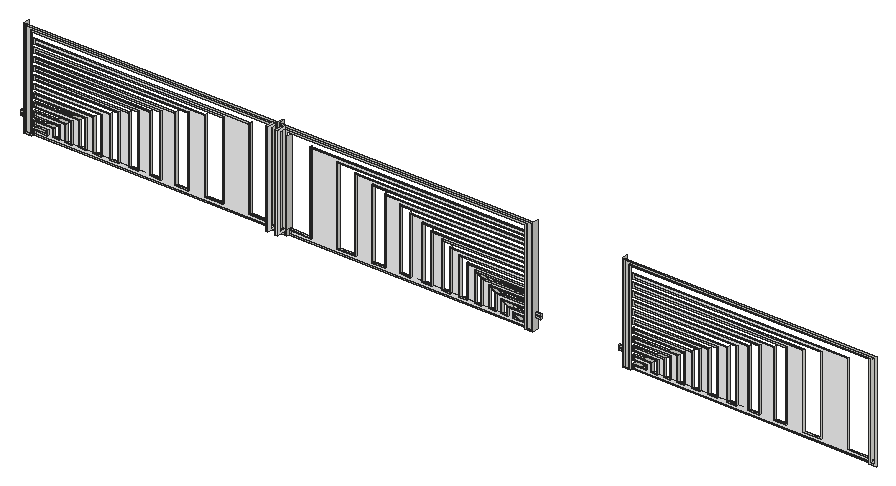
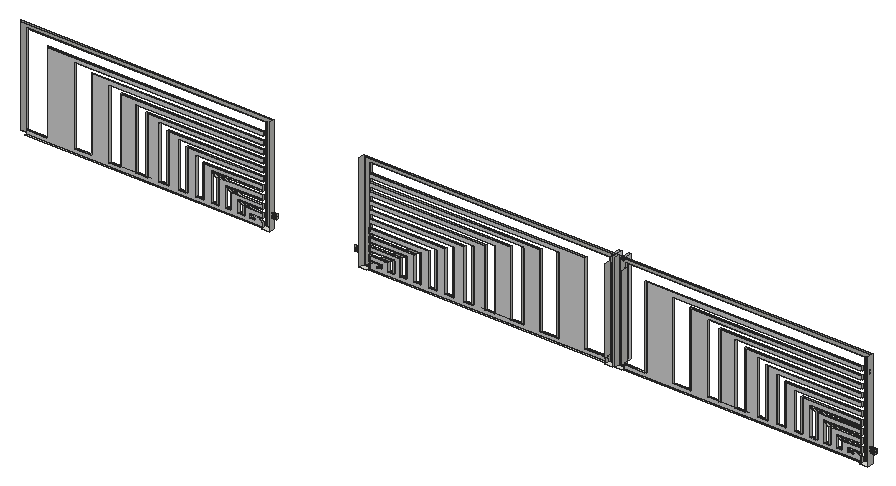
# SketchUp Ruby script. Lengths in inches.
U = 1.inch
M = Sketchup.active_model
def pt(a) = Geom::Point3d.new(a.map { |v| v * U })
def face(e, loops, mat)
  f = e.add_face(loops[0].map { |a| pt(a) })
  loops[1..].each { |l| e.add_face(l.map { |a| pt(a) }).erase! }
  f.material = f.back_material = mat if mat
  f
end
# faces: each face lists its corners as indices into pts; further lists are holes
def faces(e, pts, list, mat = nil) = list.each { |f| face(e, (f[0].is_a?(Array) ? f : [f]).map { |l| l.map { |i| pts[i] } }, mat) }
# xy, xz, yz: faces in a plane at the given z, y or x. An outline is a flat list of corners, or four numbers for a rectangle; further outlines are holes
def ring(l) = l.size == 4 ? [[l[0], l[1]], [l[2], l[1]], [l[2], l[3]], [l[0], l[3]]] : l.each_slice(2).to_a
def flat(e, list, mat, &to3) = list.each { |f| face(e, (f[0].is_a?(Array) ? f : [f]).map { |l| ring(l).map { |u, v| to3.(u, v) } }, mat) }
def xy(e, z, list, mat = nil) = flat(e, list, mat) { |x, y| [x, y, z] }
def xz(e, y, list, mat = nil) = flat(e, list, mat) { |x, z| [x, y, z] }
def yz(e, x, list, mat = nil) = flat(e, list, mat) { |y, z| [x, y, z] }
def lines(e, pts, list) = list.each { |a, b| e.add_line(pt(pts[a]), pt(pts[b])) }
# prism: a flat outline (further loops are holes) pulled along v
def prism(e, loops, v, mat = nil)
  f = face(e, loops, mat); d = Geom::Vector3d.new(v.map { |x| x * U })
  f.pushpull(f.normal.samedirection?(d) ? d.length : -d.length)
end
def box(e, o, s, mat = nil) = prism(e, [[o, [o[0] + s[0], o[1], o[2]], [o[0] + s[0], o[1] + s[1], o[2]], [o[0], o[1] + s[1], o[2]]]], [0, 0, s[2]], mat)
def at(x, y, z, deg = 0) = Geom::Transformation.translation(pt([x, y, z])) * Geom::Transformation.rotation(ORIGIN, Z_AXIS, deg.degrees)
def axes(o, x, y, z) = Geom::Transformation.new([*x, 0, *y, 0, *z, 0, *pt(o).to_a, 1])
def part(name) = M.definitions.add(name)
# library, detail: a bought-in or finely detailed component or shape, given as its bounding box
def library(name, o, s) = part(name).tap { |d| box(d.entities, o, s) }
def detail(e, o, s) = box(e.add_group.entities, o, s)
def put(e, d, t, mat = nil) = e.add_instance(d, t).tap { |i| i.material = mat if mat }
def group(e, t, mat = nil) = e.add_group.tap { |g| g.transformation = t; g.material = mat if mat }.entities
root = M.entities
M.materials.add("[Color_000]").color = [255, 255, 255]
xy(root,0,[[186.86,11.31,192.75,15.56],[371.55,11.31,377.4375,15.56],[378.67,11.31,384.5625,15.56],[563.36,11.31,569.26,15.56],[636.76,11.31,642.65,15.56],
  [192.75,12.93,371.55,14.31],[384.5625,12.93,563.36,14.31],[642.65,12.93,821.45,14.31]])
xy(root,0.49,[[193.54,12.93,370.76,13.56],[385.35,12.93,562.58,13.56],[643.44,12.93,820.67,13.56]])
xy(root,0.7,[[187.97,11.31,191.63,11.81],[372.66,11.31,376.32,11.81],[379.79,11.31,383.45,11.81],[564.48,11.31,568.14,11.81],[637.88,11.31,641.54,11.81]])
xy(root,2.12,[[373.64,4.75,375.46,11.81],[380.65,4.75,382.48,11.81]],"[Color_000]")
xy(root,3.2,[[193.54,12.93,199.38,13.56],[199.38,12.93,203.4375,13.56],[206.84,12.93,212.06,13.56],[216.11,12.93,221.45,13.56],[226.23,12.93,231.97,13.56],
  [237.375,12.93,243.66,13.56],[249.79,12.93,256.71,13.56],[263.81,12.93,271.47,13.56],[279.92,12.93,288.49,13.56],[298.9,12.93,308.95,13.56],
  [321.26,12.93,335.28,13.56],[354.73,12.93,370.76,13.56],[385.35,12.93,401.38,13.56],[420.83,12.93,434.85,13.56],[447.17,12.93,457.21,13.56],
  [467.62,12.93,476.19,13.56],[484.64,12.93,492.31,13.56],[499.4,12.93,506.32,13.56],[512.45,12.93,518.74,13.56],[524.14,12.93,529.88,13.56],
  [534.66,12.93,540,13.56],[544.05,12.93,549.28,13.56],[552.68,12.93,556.73,13.56],[556.73,12.93,562.58,13.56],[643.44,12.93,649.29,13.56],
  [649.29,12.93,653.34,13.56],[656.74,12.93,661.97,13.56],[666.01,12.93,671.36,13.56],[676.14,12.93,681.88,13.56],[687.28,12.93,693.57,13.56],
  [699.7,12.93,706.61,13.56],[713.71,12.93,721.38,13.56],[729.83,12.93,738.4,13.56],[748.81,12.93,758.85,13.56]])
xy(root,3.52,[[373.64,7.12,375.46,11.81],[380.65,7.12,382.48,11.81]],"[Color_000]")
xy(root,3.7,[[199.38,12.93,202.65,14.31],[207.625,12.93,211.27,12.93,211.27,12.97],[207.625,12.93,211.27,12.97,211.27,14.31,207.625,14.31],[216.9,12.93,220.67,12.93,220.67,13.08,216.9,13.04],[227.02,12.93,231.18,12.93,231.18,13.19,227.02,13.15],
  [238.16,12.93,242.875,12.93,242.875,13.32,238.16,13.27],[250.58,12.93,255.92,12.93,255.92,13.46,250.58,13.4],[264.59,12.93,270.68,12.93,270.68,13.62,264.59,13.55],[280.71,12.93,287.71,12.93,287.71,13.8,280.71,13.73],[299.6875,12.93,308.16,12.93,308.16,14.02,299.6875,13.93],
  [322.05,12.93,334.49,12.93,334.49,14.31,322.05,14.17],[355.52,12.93,371.55,14.31],[384.5625,12.93,400.59,14.31],[421.62,12.93,421.62,14.31,434.07,14.17,434.07,12.93],[447.95,12.93,447.95,14.02,456.42,13.93,456.42,12.93],
  [468.41,12.93,468.41,13.8,475.4,13.73,475.4,12.93],[485.43,12.93,485.43,13.62,491.52,13.55,491.52,12.93],[500.19,12.93,500.19,13.46,505.53,13.4,505.53,12.93],[513.24,12.93,513.24,13.32,517.95,13.27,517.95,12.93],[524.93,12.93,524.93,13.19,529.09,13.15,529.09,12.93],
  [535.45,12.93,535.45,13.08,539.22,13.04,539.22,12.93],[544.84,12.93,544.84,12.97,548.49,12.93],[548.49,12.93,544.84,12.97,544.84,14.31,548.49,14.31],[553.46,12.93,556.73,14.31],[649.29,12.93,652.55,14.31],
  [657.53,12.93,661.18,12.93,661.18,12.97],[657.53,12.93,661.18,12.97,661.18,14.31,657.53,14.31],[666.8,12.93,670.57,12.93,670.57,13.08,666.8,13.04],[676.92,12.93,681.09,12.93,681.09,13.19,676.92,13.15],[688.07,12.93,692.78,12.93,692.78,13.32,688.07,13.27],
  [700.48,12.93,705.83,12.93,705.83,13.46,700.48,13.4],[714.5,12.93,720.59,12.93,720.59,13.62,714.5,13.55],[730.62,12.93,737.61,12.93,737.61,13.8,730.62,13.73],[749.6,12.93,758.07,12.93,758.07,14.02,749.6,13.93],[216.9,13.04,220.67,13.08,220.67,14.31,216.9,14.31],
  [539.22,13.04,535.45,13.08,535.45,14.31,539.22,14.31],[666.8,13.04,670.57,13.08,670.57,14.31,666.8,14.31],[227.02,13.15,231.18,13.19,231.18,14.31,227.02,14.31],[529.09,13.15,524.93,13.19,524.93,14.31,529.09,14.31],[676.92,13.15,681.09,13.19,681.09,14.31,676.92,14.31],
  [238.16,13.27,242.875,13.32,242.875,14.31,238.16,14.31],[517.95,13.27,513.24,13.32,513.24,14.31,517.95,14.31],[688.07,13.27,692.78,13.32,692.78,14.31,688.07,14.31],[250.58,13.4,255.92,13.46,255.92,14.31,250.58,14.31],[505.53,13.4,500.19,13.46,500.19,14.31,505.53,14.31],
  [700.48,13.4,705.83,13.46,705.83,14.31,700.48,14.31],[264.59,13.55,270.68,13.62,270.68,14.31,264.59,14.31],[491.52,13.55,485.43,13.62,485.43,14.31,491.52,14.31],[714.5,13.55,720.59,13.62,720.59,14.31,714.5,14.31],[280.71,13.73,287.71,13.8,287.71,14.31,280.71,14.31]])
xy(root,6.12,[[192.75,12.93,196.01,14.31],[196.01,12.93,202.65,14.31],[553.46,12.93,560.1,14.31],[560.1,12.93,563.36,14.31],[642.65,12.93,645.92,14.31],
  [645.92,12.93,652.55,14.31]])
xy(root,6.62,[[193.54,12.93,196.01,13.56],[196.01,12.93,203.4375,13.56],[552.68,12.93,560.1,13.56],[560.1,12.93,562.58,13.56],[643.44,12.93,645.92,13.56],
  [645.92,12.93,653.34,13.56]])
xy(root,9.21,[[182.38,13.24,186.86,14.43],[569.26,13.24,573.73,14.43],[632.29,13.24,636.76,14.43]])
xy(root,9.32,[[193.54,12.93,199.38,13.56],[199.38,12.93,200.99,13.56],[200.99,12.93,206.84,13.56],[549.28,12.93,555.12,13.56],[555.12,12.93,556.73,13.56],
  [556.73,12.93,562.58,13.56],[643.44,12.93,649.29,13.56],[649.29,12.93,650.9,13.56],[650.9,12.93,656.74,13.56]])
xy(root,9.82,[[192.75,12.93,199.38,14.31],[199.38,12.93,200.99,14.31],[200.99,12.93,207.625,14.31],[548.49,12.93,555.12,14.31],[555.12,12.93,556.73,14.31],
  [556.73,12.93,563.36,14.31],[642.65,12.93,649.29,14.31],[649.29,12.93,650.9,14.31],[650.9,12.93,657.53,14.31]])
xy(root,10.5,[[182.38,13.24,186.86,14.43],[569.26,13.24,573.73,14.43],[632.29,13.24,636.76,14.43]])
xy(root,11.42,[[182.38,13.24,186.86,14.43],[569.26,13.24,573.73,14.43],[632.29,13.24,636.76,14.43]])
xy(root,12.24,[[192.75,12.93,204.26,14.31],[204.26,12.93,211.27,14.31],[544.84,12.93,551.85,14.31],[551.85,12.93,563.36,14.31],[642.65,12.93,654.17,14.31],
  [654.17,12.93,661.18,14.31]])
xy(root,12.71,[[182.38,13.24,186.86,14.43],[569.26,13.24,573.73,14.43],[632.29,13.24,636.76,14.43]])
xy(root,12.74,[[193.54,12.93,204.26,13.56],[204.26,12.93,212.06,13.56],[544.05,12.93,551.85,13.56],[551.85,12.93,562.58,13.56],[643.44,12.93,654.17,13.56],
  [654.17,12.93,661.97,13.56]])
xy(root,15.44,[[193.54,12.93,209.89,13.56],[209.89,12.93,216.11,13.56],[540,12.93,546.22,13.56],[546.22,12.93,562.58,13.56],[643.44,12.93,659.79,13.56],
  [659.79,12.93,666.01,13.56]])
xy(root,15.9375,[[192.75,12.93,209.89,14.31],[209.89,12.93,216.9,14.31],[539.22,12.93,546.22,14.31],[546.22,12.93,563.36,14.31],[642.65,12.93,659.79,14.31],
  [659.79,12.93,666.8,14.31]])
xy(root,18.36,[[192.75,12.93,213.58,14.31],[213.58,12.93,220.67,14.31],[535.45,12.93,542.53,14.31],[542.53,12.93,563.36,14.31],[642.65,12.93,663.48,14.31],
  [663.48,12.93,670.57,14.31]])
xy(root,18.86,[[193.54,12.93,213.58,13.56],[213.58,12.93,221.45,13.56],[534.66,12.93,542.53,13.56],[542.53,12.93,562.58,13.56],[643.44,12.93,663.48,13.56],
  [663.48,12.93,671.36,13.56]])
xy(root,21.57,[[193.54,12.93,219.5625,13.56],[219.5625,12.93,226.23,13.56],[529.88,12.93,536.55,13.56],[536.55,12.93,562.58,13.56],[643.44,12.93,669.47,13.56],
  [669.47,12.93,676.14,13.56]])
xy(root,22.06,[[192.75,12.93,219.5625,14.31],[219.5625,12.93,227.02,14.31],[529.09,12.93,536.55,14.31],[536.55,12.93,563.36,14.31],[642.65,12.93,669.47,14.31],
  [669.47,12.93,676.92,14.31]])
xy(root,24.48,[[192.75,12.93,223.73,14.31],[223.73,12.93,231.18,14.31],[524.93,12.93,532.38,14.31],[532.38,12.93,563.36,14.31],[642.65,12.93,673.64,14.31],
  [673.64,12.93,681.09,14.31]])
xy(root,24.98,[[193.54,12.93,223.73,13.56],[223.73,12.93,231.97,13.56],[524.14,12.93,532.38,13.56],[532.38,12.93,562.58,13.56],[643.44,12.93,673.64,13.56],
  [673.64,12.93,681.88,13.56]])
xz(root,4.75,[[373.64,2.12,375.46,72.7],[380.65,2.12,382.48,72.7]],"[Color_000]")
xz(root,7.12,[[373.64,3.52,375.46,71.3],[380.65,3.52,382.48,71.3]],"[Color_000]")
xz(root,11.31,[[[186.86,0,192.75,0,192.75,70.2,371.55,70.2,371.55,0,377.4375,0,377.4375,73.9,186.86,73.9],[187.97,0.7,187.97,73.2,376.32,73.2,376.32,0.7,372.66,0.7,372.66,70.9,191.63,70.9,191.63,0.7]],[[378.67,0,378.67,73.9,569.26,73.9,569.26,0,563.36,0,563.36,70.2,384.5625,70.2,384.5625,0],[379.79,0.7,383.45,0.7,383.45,70.9,564.48,70.9,564.48,0.7,568.14,0.7,568.14,73.2,379.79,73.2]],[[636.76,0,642.65,0,642.65,70.2,821.45,70.2,821.45,0,827.35,0,827.35,73.9,636.76,73.9],[637.88,0.7,637.88,73.2,826.23,73.2,826.23,0.7,822.57,0.7,822.57,70.9,641.54,70.9,641.54,0.7]]])
xz(root,11.81,[[[187.97,0.7,191.63,0.7,191.63,70.9,372.66,70.9,372.66,0.7,376.32,0.7,376.32,73.2,187.97,73.2],[373.64,71.3,375.46,72.7],[373.64,2.12,375.46,3.52]],[[379.79,0.7,379.79,73.2,568.14,73.2,568.14,0.7,564.48,0.7,564.48,70.9,383.45,70.9,383.45,0.7],[380.65,71.3,382.48,72.7],[380.65,2.12,382.48,3.52]],[[637.88,0.7,641.54,0.7,641.54,70.9,822.57,70.9,822.57,0.7,826.23,0.7,826.23,73.2,637.88,73.2],[823.54,71.3,825.37,72.7],[823.54,2.12,825.37,3.52]]])
xz(root,12.93,[[[192.75,0,371.55,0,371.55,3.7,355.52,3.7,355.52,64.91,192.75,64.91,192.75,61.21,334.49,61.21,334.49,3.7,322.05,3.7,322.05,58.79,192.75,58.79,192.75,55.09,308.16,55.09,308.16,3.7,299.6875,3.7,299.6875,52.67,192.75,52.67,192.75,48.97,287.71,48.97,287.71,3.7,280.71,3.7,280.71,46.54,192.75,46.54,192.75,42.85,270.68,42.85,270.68,3.7,264.59,3.7,264.59,40.42,192.75,40.42,192.75,36.73,255.92,36.73,255.92,3.7,250.58,3.7,250.58,34.3,192.75,34.3,192.75,30.61,242.875,30.61,242.875,3.7,238.16,3.7,238.16,28.18,192.75,28.18,192.75,24.48,231.18,24.48,231.18,3.7,227.02,3.7,227.02,22.06,192.75,22.06,192.75,18.36,220.67,18.36,220.67,3.7,216.9,3.7,216.9,15.9375,192.75,15.9375,192.75,12.24,211.27,12.24,211.27,3.7,207.625,3.7,207.625,9.82,192.75,9.82,192.75,6.12,202.65,6.12,202.65,3.7,192.75,3.7],[193.54,0.49,193.54,3.2,203.4375,3.2,203.4375,6.62,193.54,6.62,193.54,9.32,206.84,9.32,206.84,3.2,212.06,3.2,212.06,12.74,193.54,12.74,193.54,15.44,216.11,15.44,216.11,3.2,221.45,3.2,221.45,18.86,193.54,18.86,193.54,21.57,226.23,21.57,226.23,3.2,231.97,3.2,231.97,24.98,193.54,24.98,193.54,27.6875,237.375,27.6875,237.375,3.2,243.66,3.2,243.66,31.1,193.54,31.1,193.54,33.81,249.79,33.81,249.79,3.2,256.71,3.2,256.71,37.22,193.54,37.22,193.54,39.93,263.81,39.93,263.81,3.2,271.47,3.2,271.47,43.34,193.54,43.34,193.54,46.05,279.92,46.05,279.92,3.2,288.49,3.2,288.49,49.46,193.54,49.46,193.54,52.17,298.9,52.17,298.9,3.2,308.95,3.2,308.95,55.59,193.54,55.59,193.54,58.29,321.26,58.29,321.26,3.2,335.28,3.2,335.28,61.71,193.54,61.71,193.54,64.41,354.73,64.41,354.73,3.2,370.76,3.2,370.76,0.49]],[[384.5625,0,384.5625,3.7,400.59,3.7,400.59,64.91,563.36,64.91,563.36,61.21,421.62,61.21,421.62,3.7,434.07,3.7,434.07,58.79,563.36,58.79,563.36,55.09,447.95,55.09,447.95,3.7,456.42,3.7,456.42,52.67,563.36,52.67,563.36,48.97,468.41,48.97,468.41,3.7,475.4,3.7,475.4,46.54,563.36,46.54,563.36,42.85,485.43,42.85,485.43,3.7,491.52,3.7,491.52,40.42,563.36,40.42,563.36,36.73,500.19,36.73,500.19,3.7,505.53,3.7,505.53,34.3,563.36,34.3,563.36,30.61,513.24,30.61,513.24,3.7,517.95,3.7,517.95,28.18,563.36,28.18,563.36,24.48,524.93,24.48,524.93,3.7,529.09,3.7,529.09,22.06,563.36,22.06,563.36,18.36,535.45,18.36,535.45,3.7,539.22,3.7,539.22,15.9375,563.36,15.9375,563.36,12.24,544.84,12.24,544.84,3.7,548.49,3.7,548.49,9.82,563.36,9.82,563.36,6.12,553.46,6.12,553.46,3.7,563.36,3.7,563.36,0],[385.35,0.49,562.58,0.49,562.58,3.2,552.68,3.2,552.68,6.62,562.58,6.62,562.58,9.32,549.28,9.32,549.28,3.2,544.05,3.2,544.05,12.74,562.58,12.74,562.58,15.44,540,15.44,540,3.2,534.66,3.2,534.66,18.86,562.58,18.86,562.58,21.57,529.88,21.57,529.88,3.2,524.14,3.2,524.14,24.98,562.58,24.98,562.58,27.6875,518.74,27.6875,518.74,3.2,512.45,3.2,512.45,31.1,562.58,31.1,562.58,33.81,506.32,33.81,506.32,3.2,499.4,3.2,499.4,37.22,562.58,37.22,562.58,39.93,492.31,39.93,492.31,3.2,484.64,3.2,484.64,43.34,562.58,43.34,562.58,46.05,476.19,46.05,476.19,3.2,467.62,3.2,467.62,49.46,562.58,49.46,562.58,52.17,457.21,52.17,457.21,3.2,447.17,3.2,447.17,55.59,562.58,55.59,562.58,58.29,434.85,58.29,434.85,3.2,420.83,3.2,420.83,61.71,562.58,61.71,562.58,64.41,401.38,64.41,401.38,3.2,385.35,3.2]],[[642.65,0,821.45,0,821.45,3.7,805.43,3.7,805.43,64.91,642.65,64.91,642.65,61.21,784.4,61.21,784.4,3.7,771.95,3.7,771.95,58.79,642.65,58.79,642.65,55.09,758.07,55.09,758.07,3.7,749.6,3.7,749.6,52.67,642.65,52.67,642.65,48.97,737.61,48.97,737.61,3.7,730.62,3.7,730.62,46.54,642.65,46.54,642.65,42.85,720.59,42.85,720.59,3.7,714.5,3.7,714.5,40.42,642.65,40.42,642.65,36.73,705.83,36.73,705.83,3.7,700.48,3.7,700.48,34.3,642.65,34.3,642.65,30.61,692.78,30.61,692.78,3.7,688.07,3.7,688.07,28.18,642.65,28.18,642.65,24.48,681.09,24.48,681.09,3.7,676.92,3.7,676.92,22.06,642.65,22.06,642.65,18.36,670.57,18.36,670.57,3.7,666.8,3.7,666.8,15.9375,642.65,15.9375,642.65,12.24,661.18,12.24,661.18,3.7,657.53,3.7,657.53,9.82,642.65,9.82,642.65,6.12,652.55,6.12,652.55,3.7,642.65,3.7],[643.44,0.49,643.44,3.2,653.34,3.2,653.34,6.62,643.44,6.62,643.44,9.32,656.74,9.32,656.74,3.2,661.97,3.2,661.97,12.74,643.44,12.74,643.44,15.44,666.01,15.44,666.01,3.2,671.36,3.2,671.36,18.86,643.44,18.86,643.44,21.57,676.14,21.57,676.14,3.2,681.88,3.2,681.88,24.98,643.44,24.98,643.44,27.6875,687.28,27.6875,687.28,3.2,693.57,3.2,693.57,31.1,643.44,31.1,643.44,33.81,699.7,33.81,699.7,3.2,706.61,3.2,706.61,37.22,643.44,37.22,643.44,39.93,713.71,39.93,713.71,3.2,721.38,3.2,721.38,43.34,643.44,43.34,643.44,46.05,729.83,46.05,729.83,3.2,738.4,3.2,738.4,49.46,643.44,49.46,643.44,52.17,748.81,52.17,748.81,3.2,758.85,3.2,758.85,55.59,643.44,55.59,643.44,58.29,771.16,58.29,771.16,3.2,785.19,3.2,785.19,61.71,643.44,61.71,643.44,64.41,804.64,64.41,804.64,3.2,820.67,3.2,820.67,0.49]],[192.75,3.7,199.38,3.7,202.65,6.12,196.01,6.12],[556.73,3.7,553.46,6.12,560.1,6.12,563.36,3.7],
  [642.65,3.7,649.29,3.7,652.55,6.12,645.92,6.12],[200.99,9.82,207.625,9.82,207.95,10.06,211.27,12.24,204.26,12.24,204.18,12.18],[548.49,9.82,548.16,10.06,544.84,12.24,551.85,12.24,551.9375,12.18,555.12,9.82],[650.9,9.82,657.53,9.82,657.85,10.06,661.18,12.24,654.17,12.24,654.08,12.18],[209.89,15.9375,216.9,15.9375,219.96,17.95,220.67,18.36,213.58,18.36],
  [539.22,15.9375,536.15,17.95,535.45,18.36,542.53,18.36,546.22,15.9375],[659.79,15.9375,666.8,15.9375,669.87,17.95,670.57,18.36,663.48,18.36],[219.5625,22.06,227.02,22.06,231.18,24.48,223.73,24.48],[529.09,22.06,524.93,24.48,532.38,24.48,536.55,22.06],[669.47,22.06,676.92,22.06,681.09,24.48,673.64,24.48]])
xz(root,13.24,[[182.38,9.21,186.86,10.5],[569.26,9.21,573.73,10.5],[632.29,9.21,636.76,10.5],[182.38,11.42,186.86,12.71],[569.26,11.42,573.73,12.71],
  [632.29,11.42,636.76,12.71]])
xz(root,13.56,[[193.54,0.49,370.76,0.49,370.76,3.2,354.73,3.2,354.73,64.41,193.54,64.41,193.54,61.71,335.28,61.71,335.28,3.2,321.26,3.2,321.26,58.29,193.54,58.29,193.54,55.59,308.95,55.59,308.95,3.2,298.9,3.2,298.9,52.17,193.54,52.17,193.54,49.46,288.49,49.46,288.49,3.2,279.92,3.2,279.92,46.05,193.54,46.05,193.54,43.34,271.47,43.34,271.47,3.2,263.81,3.2,263.81,39.93,193.54,39.93,193.54,37.22,256.71,37.22,256.71,3.2,249.79,3.2,249.79,33.81,193.54,33.81,193.54,31.1,243.66,31.1,243.66,3.2,237.375,3.2,237.375,27.6875,193.54,27.6875,193.54,24.98,231.97,24.98,231.97,3.2,226.23,3.2,226.23,21.57,193.54,21.57,193.54,18.86,221.45,18.86,221.45,3.2,216.11,3.2,216.11,15.44,193.54,15.44,193.54,12.74,212.06,12.74,212.06,3.2,206.84,3.2,206.84,9.32,193.54,9.32,193.54,6.62,203.4375,6.62,203.4375,3.2,193.54,3.2],[385.35,0.49,385.35,3.2,401.38,3.2,401.38,64.41,562.58,64.41,562.58,61.71,420.83,61.71,420.83,3.2,434.85,3.2,434.85,58.29,562.58,58.29,562.58,55.59,447.17,55.59,447.17,3.2,457.21,3.2,457.21,52.17,562.58,52.17,562.58,49.46,467.62,49.46,467.62,3.2,476.19,3.2,476.19,46.05,562.58,46.05,562.58,43.34,484.64,43.34,484.64,3.2,492.31,3.2,492.31,39.93,562.58,39.93,562.58,37.22,499.4,37.22,499.4,3.2,506.32,3.2,506.32,33.81,562.58,33.81,562.58,31.1,512.45,31.1,512.45,3.2,518.74,3.2,518.74,27.6875,562.58,27.6875,562.58,24.98,524.14,24.98,524.14,3.2,529.88,3.2,529.88,21.57,562.58,21.57,562.58,18.86,534.66,18.86,534.66,3.2,540,3.2,540,15.44,562.58,15.44,562.58,12.74,544.05,12.74,544.05,3.2,549.28,3.2,549.28,9.32,562.58,9.32,562.58,6.62,552.68,6.62,552.68,3.2,562.58,3.2,562.58,0.49],[643.44,0.49,820.67,0.49,820.67,3.2,804.64,3.2,804.64,64.41,643.44,64.41,643.44,61.71,785.19,61.71,785.19,3.2,771.16,3.2,771.16,58.29,643.44,58.29,643.44,55.59,758.85,55.59,758.85,3.2,748.81,3.2,748.81,52.17,643.44,52.17,643.44,49.46,738.4,49.46,738.4,3.2,729.83,3.2,729.83,46.05,643.44,46.05,643.44,43.34,721.38,43.34,721.38,3.2,713.71,3.2,713.71,39.93,643.44,39.93,643.44,37.22,706.61,37.22,706.61,3.2,699.7,3.2,699.7,33.81,643.44,33.81,643.44,31.1,693.57,31.1,693.57,3.2,687.28,3.2,687.28,27.6875,643.44,27.6875,643.44,24.98,681.88,24.98,681.88,3.2,676.14,3.2,676.14,21.57,643.44,21.57,643.44,18.86,671.36,18.86,671.36,3.2,666.01,3.2,666.01,15.44,643.44,15.44,643.44,12.74,661.97,12.74,661.97,3.2,656.74,3.2,656.74,9.32,643.44,9.32,643.44,6.62,653.34,6.62,653.34,3.2,643.44,3.2]],"[Color_000]")
xz(root,13.81,[[193.54,0.49,193.54,3.52,196.38,5.63,200.95,5.63,197.6875,3.2,203.4375,3.2,203.4375,6.62,193.54,6.62,193.54,9.32,206.84,9.32,206.84,3.2,212.06,3.2,212.06,12.74,193.54,12.74,193.54,15.44,216.11,15.44,216.11,3.2,221.45,3.2,221.45,18.86,193.54,18.86,193.54,21.57,226.23,21.57,226.23,3.2,231.97,3.2,231.97,24.98,193.54,24.98,193.54,27.6875,237.375,27.6875,237.375,3.2,243.66,3.2,243.66,31.1,193.54,31.1,193.54,33.81,249.79,33.81,249.79,3.2,256.71,3.2,256.71,37.22,193.54,37.22,193.54,39.93,263.81,39.93,263.81,3.2,271.47,3.2,271.47,43.34,193.54,43.34,193.54,46.05,279.92,46.05,279.92,3.2,288.49,3.2,288.49,49.46,193.54,49.46,193.54,52.17,298.9,52.17,298.9,3.2,308.95,3.2,308.95,55.59,193.54,55.59,193.54,58.29,321.26,58.29,321.26,3.2,335.28,3.2,335.28,61.71,193.54,61.71,193.54,64.41,354.73,64.41,354.73,3.2,370.76,3.2,370.76,0.49],[385.35,0.49,562.58,0.49,562.58,3.52,559.73,5.63,555.16,5.63,558.43,3.2,552.68,3.2,552.68,6.62,562.58,6.62,562.58,9.32,549.28,9.32,549.28,3.2,544.05,3.2,544.05,12.74,562.58,12.74,562.58,15.44,540,15.44,540,3.2,534.66,3.2,534.66,18.86,562.58,18.86,562.58,21.57,529.88,21.57,529.88,3.2,524.14,3.2,524.14,24.98,562.58,24.98,562.58,27.6875,518.74,27.6875,518.74,3.2,512.45,3.2,512.45,31.1,562.58,31.1,562.58,33.81,506.32,33.81,506.32,3.2,499.4,3.2,499.4,37.22,562.58,37.22,562.58,39.93,492.31,39.93,492.31,3.2,484.64,3.2,484.64,43.34,562.58,43.34,562.58,46.05,476.19,46.05,476.19,3.2,467.62,3.2,467.62,49.46,562.58,49.46,562.58,52.17,457.21,52.17,457.21,3.2,447.17,3.2,447.17,55.59,562.58,55.59,562.58,58.29,434.85,58.29,434.85,3.2,420.83,3.2,420.83,61.71,562.58,61.71,562.58,64.41,401.38,64.41,401.38,3.2,385.35,3.2],[643.44,0.49,643.44,3.52,646.29,5.63,650.86,5.63,647.59,3.2,653.34,3.2,653.34,6.62,643.44,6.62,643.44,9.32,656.74,9.32,656.74,3.2,661.97,3.2,661.97,12.74,643.44,12.74,643.44,15.44,666.01,15.44,666.01,3.2,671.36,3.2,671.36,18.86,643.44,18.86,643.44,21.57,676.14,21.57,676.14,3.2,681.88,3.2,681.88,24.98,643.44,24.98,643.44,27.6875,687.28,27.6875,687.28,3.2,693.57,3.2,693.57,31.1,643.44,31.1,643.44,33.81,699.7,33.81,699.7,3.2,706.61,3.2,706.61,37.22,643.44,37.22,643.44,39.93,713.71,39.93,713.71,3.2,721.38,3.2,721.38,43.34,643.44,43.34,643.44,46.05,729.83,46.05,729.83,3.2,738.4,3.2,738.4,49.46,643.44,49.46,643.44,52.17,748.81,52.17,748.81,3.2,758.85,3.2,758.85,55.59,643.44,55.59,643.44,58.29,771.16,58.29,771.16,3.2,785.19,3.2,785.19,61.71,643.44,61.71,643.44,64.41,804.64,64.41,804.64,3.2,820.67,3.2,820.67,0.49]],"[Color_000]")
yz(root,182.38,[[13.24,9.21,14.43,10.5],[13.24,11.42,14.43,12.71]])
yz(root,186.86,[[[11.31,0,15.56,73.9],[13.24,63.67,14.43,64.96],[13.24,61.46,14.43,62.75],[13.24,11.42,14.43,12.71],[13.24,9.21,14.43,10.5]]])
yz(root,187.97,[[11.31,0.7,11.81,73.2]])
yz(root,191.63,[[11.31,0.7,11.81,70.9]])
yz(root,192.75,[[12.93,0,14.31,3.7],[12.93,6.12,14.31,9.82],[12.93,12.24,14.31,15.9375],[12.93,18.36,14.31,22.06],[12.93,24.48,14.31,28.18]])
yz(root,193.54,[[12.93,0.49,13.56,3.2],[12.93,6.62,13.56,9.32],[12.93,12.74,13.56,15.44],[12.93,18.86,13.56,21.57],[12.93,24.98,13.56,27.6875]])
yz(root,202.65,[[12.93,3.7,14.31,6.12]])
yz(root,203.4375,[[12.93,3.2,13.56,6.62]])
yz(root,206.84,[[12.93,3.2,13.56,9.32]])
yz(root,207.625,[[12.93,3.7,14.31,9.82]])
yz(root,211.27,[[12.93,3.7,14.31,12.24]])
yz(root,212.06,[[12.93,3.2,13.56,12.74]])
yz(root,216.11,[[12.93,3.2,13.56,15.44]])
yz(root,216.9,[[12.93,3.7,14.31,15.9375]])
yz(root,220.67,[[12.93,3.7,14.31,18.36]])
yz(root,221.45,[[12.93,3.2,13.56,18.86]])
yz(root,226.23,[[12.93,3.2,13.56,21.57]])
yz(root,227.02,[[12.93,3.7,14.31,22.06]])
yz(root,231.18,[[12.93,3.7,14.31,24.48]])
yz(root,231.97,[[12.93,3.2,13.56,24.98]])
yz(root,237.375,[[12.93,3.2,13.56,27.6875]])
yz(root,238.16,[[12.93,3.7,14.31,28.18]])
yz(root,242.875,[[12.93,3.7,14.31,30.61]])
yz(root,243.66,[[12.93,3.2,13.56,31.1]])
yz(root,249.79,[[12.93,3.2,13.56,33.81]])
yz(root,250.58,[[12.93,3.7,14.31,34.3]])
yz(root,255.92,[[12.93,3.7,14.31,36.73]])
yz(root,256.71,[[12.93,3.2,13.56,37.22]])
yz(root,263.81,[[12.93,3.2,13.56,39.93]])
yz(root,264.59,[[12.93,3.7,14.31,40.42]])
yz(root,270.68,[[12.93,3.7,14.31,42.85]])
yz(root,271.47,[[12.93,3.2,13.56,43.34]])
yz(root,279.92,[[12.93,3.2,13.56,46.05]])
yz(root,280.71,[[12.93,3.7,14.31,46.54]])
yz(root,287.71,[[12.93,3.7,14.31,48.97]])
yz(root,288.49,[[12.93,3.2,13.56,49.46]])
yz(root,298.9,[[12.93,3.2,13.56,52.17]])
yz(root,299.6875,[[12.93,3.7,14.31,52.67]])
yz(root,308.16,[[12.93,3.7,14.31,55.09]])
yz(root,308.95,[[12.93,3.2,13.56,55.59]])
yz(root,321.26,[[12.93,3.2,13.56,58.29]])
yz(root,322.05,[[12.93,3.7,14.31,58.6]])
yz(root,334.49,[[12.93,3.7,14.31,61.21]])
yz(root,335.28,[[12.93,3.2,13.56,61.71]])
yz(root,354.73,[[12.93,3.2,13.56,64.41]])
yz(root,355.52,[[12.93,3.7,14.31,64.91]])
yz(root,370.76,[[12.93,0.49,13.56,3.2]])
yz(root,371.55,[[11.31,0,12.93,3.7],[12.93,0,14.31,3.7],[11.31,3.7,15.56,66.96]])
yz(root,372.66,[[11.31,0.7,11.81,3.7],[11.31,3.7,11.81,66.96]])
yz(root,373.64,[[4.75,2.12,4.75,72.7,11.81,72.7,11.81,71.3,7.12,71.3,7.12,3.52,11.81,3.52,11.81,2.12]],"[Color_000]")
yz(root,375.46,[[4.75,2.12,11.81,2.12,11.81,3.52,7.12,3.52,7.12,71.3,11.81,71.3,11.81,72.7,4.75,72.7]],"[Color_000]")
yz(root,376.32,[[11.31,0.7,11.81,73.2]])
yz(root,377.4375,[[11.31,0,15.56,73.9]])
yz(root,378.67,[[11.31,0,15.56,73.9]])
yz(root,379.79,[[11.31,0.7,11.81,73.2]])
yz(root,380.65,[[4.75,2.12,11.81,2.12,11.81,3.52,7.12,3.52,7.12,71.3,11.81,71.3,11.81,72.7,4.75,72.7]],"[Color_000]")
yz(root,382.48,[[4.75,2.12,4.75,72.7,11.81,72.7,11.81,71.3,7.12,71.3,7.12,3.52,11.81,3.52,11.81,2.12]],"[Color_000]")
yz(root,383.45,[[11.31,0.7,11.81,3.7],[11.31,3.7,11.81,66.96]])
yz(root,384.5625,[[11.31,0,12.93,3.7],[12.93,0,14.31,3.7],[11.31,3.7,15.56,66.96]])
yz(root,385.35,[[12.93,0.49,13.56,3.2]])
yz(root,400.59,[[12.93,3.7,14.31,64.91]])
yz(root,401.38,[[12.93,3.2,13.56,64.41]])
yz(root,420.83,[[12.93,3.2,13.56,61.71]])
yz(root,421.62,[[12.93,3.7,14.31,61.21]])
yz(root,434.07,[[12.93,3.7,14.31,58.6]])
yz(root,434.85,[[12.93,3.2,13.56,58.29]])
yz(root,447.17,[[12.93,3.2,13.56,55.59]])
yz(root,447.95,[[12.93,3.7,14.31,55.09]])
yz(root,456.42,[[12.93,3.7,14.31,52.67]])
yz(root,457.21,[[12.93,3.2,13.56,52.17]])
yz(root,467.62,[[12.93,3.2,13.56,49.46]])
yz(root,468.41,[[12.93,3.7,14.31,48.97]])
yz(root,475.4,[[12.93,3.7,14.31,46.54]])
yz(root,476.19,[[12.93,3.2,13.56,46.05]])
yz(root,484.64,[[12.93,3.2,13.56,43.34]])
yz(root,485.43,[[12.93,3.7,14.31,42.85]])
yz(root,491.52,[[12.93,3.7,14.31,40.42]])
yz(root,492.31,[[12.93,3.2,13.56,39.93]])
yz(root,499.4,[[12.93,3.2,13.56,37.22]])
yz(root,500.19,[[12.93,3.7,14.31,36.73]])
yz(root,505.53,[[12.93,3.7,14.31,34.3]])
yz(root,506.32,[[12.93,3.2,13.56,33.81]])
yz(root,512.45,[[12.93,3.2,13.56,31.1]])
yz(root,513.24,[[12.93,3.7,14.31,30.61]])
yz(root,517.95,[[12.93,3.7,14.31,28.18]])
yz(root,518.74,[[12.93,3.2,13.56,27.6875]])
yz(root,524.14,[[12.93,3.2,13.56,24.98]])
yz(root,524.93,[[12.93,3.7,14.31,24.48]])
yz(root,529.09,[[12.93,3.7,14.31,22.06]])
yz(root,529.88,[[12.93,3.2,13.56,21.57]])
yz(root,534.66,[[12.93,3.2,13.56,18.86]])
yz(root,535.45,[[12.93,3.7,14.31,18.36]])
yz(root,539.22,[[12.93,3.7,14.31,15.9375]])
yz(root,540,[[12.93,3.2,13.56,15.44]])
yz(root,544.05,[[12.93,3.2,13.56,12.74]])
yz(root,544.84,[[12.93,3.7,14.31,12.24]])
yz(root,548.49,[[12.93,3.7,14.31,9.82]])
yz(root,549.28,[[12.93,3.2,13.56,9.32]])
yz(root,552.68,[[12.93,3.2,13.56,6.62]])
yz(root,553.46,[[12.93,3.7,14.31,6.12]])
yz(root,562.58,[[12.93,0.49,13.56,3.2],[12.93,6.62,13.56,9.32],[12.93,12.74,13.56,15.44],[12.93,18.86,13.56,21.57],[12.93,24.98,13.56,27.6875]])
yz(root,563.36,[[12.93,0,14.31,3.7],[12.93,6.12,14.31,9.82],[12.93,12.24,14.31,15.9375],[12.93,18.36,14.31,22.06],[12.93,24.48,14.31,28.18]])
yz(root,564.48,[[11.31,0.7,11.81,70.9]])
yz(root,568.14,[[11.31,0.7,11.81,73.2]])
yz(root,569.26,[[[11.31,0,15.56,73.9],[13.24,63.67,14.43,64.96],[13.24,61.46,14.43,62.75],[13.24,11.42,14.43,12.71],[13.24,9.21,14.43,10.5]]])
yz(root,573.73,[[13.24,9.21,14.43,10.5],[13.24,11.42,14.43,12.71]])
yz(root,632.29,[[13.24,9.21,14.43,10.5],[13.24,11.42,14.43,12.71]])
yz(root,636.76,[[[11.31,0,15.56,73.9],[13.24,63.67,14.43,64.96],[13.24,61.46,14.43,62.75],[13.24,11.42,14.43,12.71],[13.24,9.21,14.43,10.5]]])
yz(root,637.88,[[11.31,0.7,11.81,73.2]])
yz(root,641.54,[[11.31,0.7,11.81,70.9]])
yz(root,642.65,[[12.93,0,14.31,3.7],[12.93,6.12,14.31,9.82],[12.93,12.24,14.31,15.9375],[12.93,18.36,14.31,22.06],[12.93,24.48,14.31,28.18]])
yz(root,643.44,[[12.93,0.49,13.56,3.2],[12.93,6.62,13.56,9.32],[12.93,12.74,13.56,15.44],[12.93,18.86,13.56,21.57],[12.93,24.98,13.56,27.6875]])
yz(root,652.55,[[12.93,3.7,14.31,6.12]])
yz(root,653.34,[[12.93,3.2,13.56,6.62]])
yz(root,656.74,[[12.93,3.2,13.56,9.32]])
yz(root,657.53,[[12.93,3.7,14.31,9.82]])
yz(root,661.18,[[12.93,3.7,14.31,12.24]])
yz(root,661.97,[[12.93,3.2,13.56,12.74]])
yz(root,666.01,[[12.93,3.2,13.56,15.44]])
yz(root,666.8,[[12.93,3.7,14.31,15.9375]])
yz(root,670.57,[[12.93,3.7,14.31,18.36]])
yz(root,671.36,[[12.93,3.2,13.56,18.86]])
yz(root,676.14,[[12.93,3.2,13.56,21.57]])
yz(root,676.92,[[12.93,3.7,14.31,22.06]])
yz(root,681.09,[[12.93,3.7,14.31,24.48]])
yz(root,681.88,[[12.93,3.2,13.56,24.98]])
yz(root,687.28,[[12.93,3.2,13.56,27.6875]])
yz(root,688.07,[[12.93,3.7,14.31,28.18]])
yz(root,692.78,[[12.93,3.7,14.31,30.61]])
yz(root,693.57,[[12.93,3.2,13.56,31.1]])
yz(root,699.7,[[12.93,3.2,13.56,33.81]])
yz(root,700.48,[[12.93,3.7,14.31,34.3]])
yz(root,705.83,[[12.93,3.7,14.31,36.73]])
yz(root,706.61,[[12.93,3.2,13.56,37.22]])
yz(root,713.71,[[12.93,3.2,13.56,39.93]])
yz(root,714.5,[[12.93,3.7,14.31,40.42]])
yz(root,720.59,[[12.93,3.7,14.31,42.85]])
yz(root,721.38,[[12.93,3.2,13.56,43.34]])
yz(root,729.83,[[12.93,3.2,13.56,46.05]])
yz(root,730.62,[[12.93,3.7,14.31,46.54]])
yz(root,737.61,[[12.93,3.7,14.31,48.97]])
yz(root,738.4,[[12.93,3.2,13.56,49.46]])
yz(root,748.81,[[12.93,3.2,13.56,52.17]])
yz(root,749.6,[[12.93,3.7,14.31,52.67]])
yz(root,758.07,[[12.93,3.7,14.31,55.09]])
p = [[196.01,14.31,6.12],[192.75,14.31,3.7],[192.75,12.93,3.7],[196.01,12.93,6.12],[199.38,14.31,3.7],[202.65,14.31,6.12],
  [202.65,12.93,6.12],[199.38,12.93,3.7],[556.73,14.31,3.7],[553.46,14.31,6.12],[553.46,12.93,6.12],[556.73,12.93,3.7],
  [560.1,14.31,6.12],[563.36,14.31,3.7],[563.36,12.93,3.7],[560.1,12.93,6.12],[645.92,14.31,6.12],[642.65,14.31,3.7],
  [642.65,12.93,3.7],[645.92,12.93,6.12],[649.29,14.31,3.7],[652.55,14.31,6.12],[652.55,12.93,6.12],[649.29,12.93,3.7],
  [204.18,14.31,12.18],[200.99,14.31,9.82],[200.99,12.93,9.82],[204.18,12.93,12.18],[207.625,14.31,9.82],[207.95,14.31,10.06],
  [207.95,12.93,10.06],[207.625,12.93,9.82],[548.49,14.31,9.82],[548.16,14.31,10.06],[548.16,12.93,10.06],[548.49,12.93,9.82],
  [551.9375,14.31,12.18],[555.12,14.31,9.82],[555.12,12.93,9.82],[551.9375,12.93,12.18],[654.08,14.31,12.18],[650.9,14.31,9.82],
  [650.9,12.93,9.82],[654.08,12.93,12.18],[657.53,14.31,9.82],[657.85,14.31,10.06],[657.85,12.93,10.06],[657.53,12.93,9.82],
  [211.27,14.31,12.24],[211.27,12.93,12.24],[544.84,14.31,12.24],[544.84,12.93,12.24],[661.18,14.31,12.24],[661.18,12.93,12.24],
  [204.26,14.31,12.24],[204.26,12.93,12.24],[551.85,14.31,12.24],[551.85,12.93,12.24],[654.17,14.31,12.24],[654.17,12.93,12.24],
  [213.58,14.31,18.36],[209.89,14.31,15.9375],[209.89,12.93,15.9375],[213.58,12.93,18.36],[216.9,14.31,15.9375],[219.96,14.31,17.95],
  [219.96,12.93,17.95],[216.9,12.93,15.9375],[539.22,14.31,15.9375],[536.15,14.31,17.95],[536.15,12.93,17.95],[539.22,12.93,15.9375],
  [542.53,14.31,18.36],[546.22,14.31,15.9375],[546.22,12.93,15.9375],[542.53,12.93,18.36],[663.48,14.31,18.36],[659.79,14.31,15.9375],
  [659.79,12.93,15.9375],[663.48,12.93,18.36],[666.8,14.31,15.9375],[669.87,14.31,17.95],[669.87,12.93,17.95],[666.8,12.93,15.9375],
  [220.67,14.31,18.36],[220.67,12.93,18.36],[535.45,14.31,18.36],[535.45,12.93,18.36],[670.57,14.31,18.36],[670.57,12.93,18.36],
  [223.73,14.31,24.48],[219.5625,14.31,22.06],[219.5625,12.93,22.06],[223.73,12.93,24.48],[227.02,14.31,22.06],[231.18,14.31,24.48],
  [231.18,12.93,24.48],[227.02,12.93,22.06],[529.09,14.31,22.06],[524.93,14.31,24.48],[524.93,12.93,24.48],[529.09,12.93,22.06],
  [532.38,14.31,24.48],[536.55,14.31,22.06],[536.55,12.93,22.06],[532.38,12.93,24.48],[673.64,14.31,24.48],[669.47,14.31,22.06],
  [669.47,12.93,22.06],[673.64,12.93,24.48],[676.92,14.31,22.06],[681.09,14.31,24.48],[681.09,12.93,24.48],[676.92,12.93,22.06],
  [517.95,13.27,3.7],[524.93,13.19,3.7],[505.53,13.4,3.7],[513.24,13.32,3.7],[491.52,13.55,3.7],[500.19,13.46,3.7],
  [539.22,13.04,3.7],[544.84,12.97,3.7],[475.4,13.73,3.7],[485.43,13.62,3.7],[529.09,13.15,3.7],[535.45,13.08,3.7],
  [456.42,13.93,3.7],[468.41,13.8,3.7],[238.16,13.27,3.7],[231.18,13.19,3.7],[250.58,13.4,3.7],[242.875,13.32,3.7],
  [264.59,13.55,3.7],[255.92,13.46,3.7],[216.9,13.04,3.7],[211.27,12.97,3.7],[280.71,13.73,3.7],[270.68,13.62,3.7],
  [227.02,13.15,3.7],[220.67,13.08,3.7],[299.6875,13.93,3.7],[287.71,13.8,3.7],[688.07,13.27,3.7],[681.09,13.19,3.7],
  [700.48,13.4,3.7],[692.78,13.32,3.7],[714.5,13.55,3.7],[705.83,13.46,3.7],[666.8,13.04,3.7],[661.18,12.97,3.7],
  [730.62,13.73,3.7],[720.59,13.62,3.7],[676.92,13.15,3.7],[670.57,13.08,3.7],[749.6,13.93,3.7],[737.61,13.8,3.7]]
faces(root,p,[[0,1,2,3],[4,5,6,7],[8,9,10,11],[12,13,14,15],[16,17,18,19],[20,21,22,23],[24,25,26,27],[28,29,30,31],
  [32,33,34,35],[36,37,38,39],[40,41,42,43],[44,45,46,47],[29,48,49,30],[33,50,51,34],[45,52,53,46],[54,24,27,55],
  [56,36,39,57],[58,40,43,59],[60,61,62,63],[64,65,66,67],[68,69,70,71],[72,73,74,75],[76,77,78,79],[80,81,82,83],
  [65,84,85,66],[69,86,87,70],[81,88,89,82],[90,91,92,93],[94,95,96,97],[98,99,100,101],[102,103,104,105],[106,107,108,109],
  [110,111,112,113]])
lines(root,p,[[114,115],[116,117],[118,119],[120,121],[122,123],[124,125],[126,127],[128,129],[130,131],[132,133],[134,135],[136,137],
  [138,139],[140,141],[142,143],[144,145],[146,147],[148,149],[150,151],[152,153],[154,155]])
